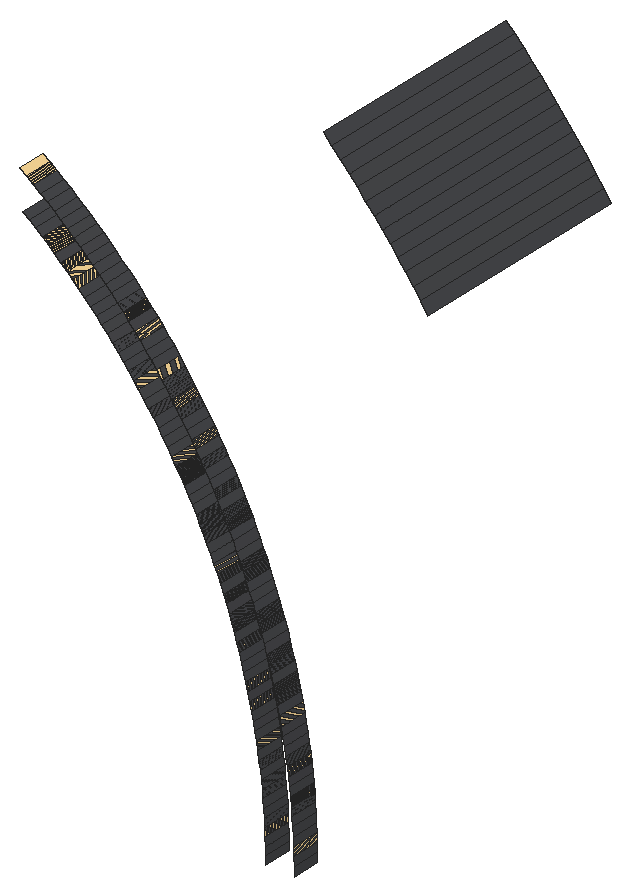
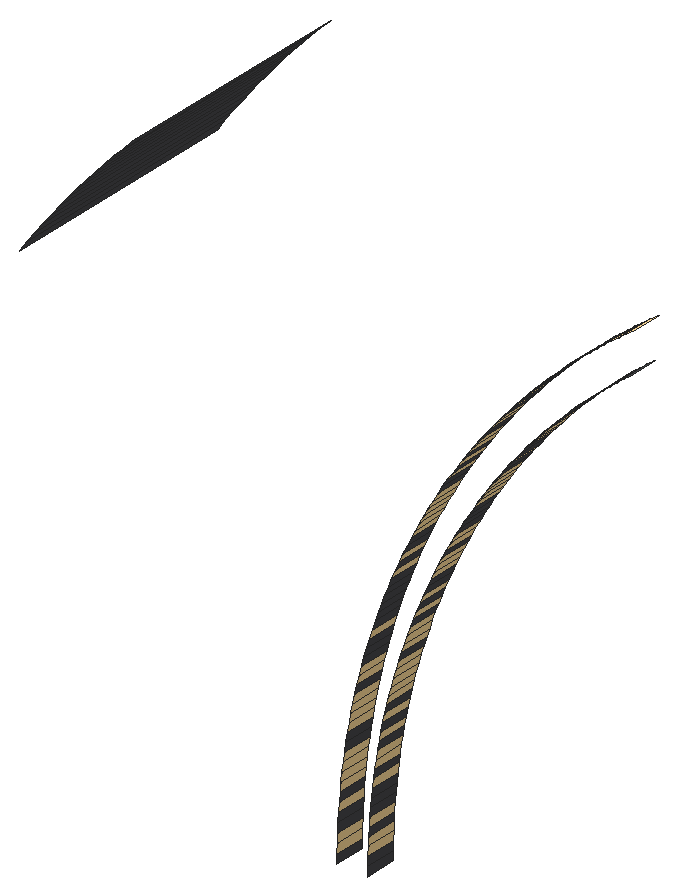
# SketchUp Ruby script. Lengths in inches.
U = 1.inch
M = Sketchup.active_model
def pt(a) = Geom::Point3d.new(a.map { |v| v * U })
def face(e, loops, mat)
  f = e.add_face(loops[0].map { |a| pt(a) })
  loops[1..].each { |l| e.add_face(l.map { |a| pt(a) }).erase! }
  f.material = f.back_material = mat if mat
  f
end
# faces: each face lists its corners as indices into pts; further lists are holes
def faces(e, pts, list, mat = nil) = list.each { |f| face(e, (f[0].is_a?(Array) ? f : [f]).map { |l| l.map { |i| pts[i] } }, mat) }
# xy, xz, yz: faces in a plane at the given z, y or x. An outline is a flat list of corners, or four numbers for a rectangle; further outlines are holes
def ring(l) = l.size == 4 ? [[l[0], l[1]], [l[2], l[1]], [l[2], l[3]], [l[0], l[3]]] : l.each_slice(2).to_a
def flat(e, list, mat, &to3) = list.each { |f| face(e, (f[0].is_a?(Array) ? f : [f]).map { |l| ring(l).map { |u, v| to3.(u, v) } }, mat) }
def xy(e, z, list, mat = nil) = flat(e, list, mat) { |x, y| [x, y, z] }
def xz(e, y, list, mat = nil) = flat(e, list, mat) { |x, z| [x, y, z] }
def yz(e, x, list, mat = nil) = flat(e, list, mat) { |y, z| [x, y, z] }
def lines(e, pts, list) = list.each { |a, b| e.add_line(pt(pts[a]), pt(pts[b])) }
# prism: a flat outline (further loops are holes) pulled along v
def prism(e, loops, v, mat = nil)
  f = face(e, loops, mat); d = Geom::Vector3d.new(v.map { |x| x * U })
  f.pushpull(f.normal.samedirection?(d) ? d.length : -d.length)
end
def box(e, o, s, mat = nil) = prism(e, [[o, [o[0] + s[0], o[1], o[2]], [o[0] + s[0], o[1] + s[1], o[2]], [o[0], o[1] + s[1], o[2]]]], [0, 0, s[2]], mat)
def at(x, y, z, deg = 0) = Geom::Transformation.translation(pt([x, y, z])) * Geom::Transformation.rotation(ORIGIN, Z_AXIS, deg.degrees)
def axes(o, x, y, z) = Geom::Transformation.new([*x, 0, *y, 0, *z, 0, *pt(o).to_a, 1])
def part(name) = M.definitions.add(name)
# library, detail: a bought-in or finely detailed component or shape, given as its bounding box
def library(name, o, s) = part(name).tap { |d| box(d.entities, o, s) }
def detail(e, o, s) = box(e.add_group.entities, o, s)
def put(e, d, t, mat = nil) = e.add_instance(d, t).tap { |i| i.material = mat if mat }
def group(e, t, mat = nil) = e.add_group.tap { |g| g.transformation = t; g.material = mat if mat }.entities
root = M.entities
M.materials.add("1432 AP 8245 TAR ROAD").color = [71, 72, 75]
M.materials.add("Outer Light").color = [251, 217, 152]
yz(root,426.5,[[95.37,410.79,96.87,411.23]],"1432 AP 8245 TAR ROAD")
yz(root,426.5,[[95.37,410.79,96.87,411.23]],"Outer Light")
yz(root,428,[[95.37,410.79,96.87,411.25]],"1432 AP 8245 TAR ROAD")
yz(root,428,[[95.37,410.79,96.87,411.25]],"Outer Light")
p = [[426.49,95.37,411.67],[426.5,95.37,411.23],[426.5,96.87,411.23],[426.49,96.87,411.67],[426.49,96.87,411.67],[426.5,96.87,411.23],
  [426.5,95.37,411.23],[426.49,95.37,411.67],[428,96.87,411.25],[427.99,96.87,411.71],[427.99,95.37,411.71],[428,95.37,411.25],
  [428,95.37,411.25],[427.99,95.37,411.71],[427.99,96.87,411.71],[428,96.87,411.25],[426.47,95.37,412.11],[426.47,96.87,412.11],
  [426.47,96.87,412.11],[426.47,95.37,412.11],[427.97,96.87,412.17],[427.97,95.37,412.17],[427.97,95.37,412.17],[427.97,96.87,412.17],
  [426.45,95.37,412.55],[426.45,96.87,412.55],[426.45,96.87,412.55],[426.45,95.37,412.55],[427.95,96.87,412.625],[427.95,95.37,412.625],
  [427.95,95.37,412.625],[427.95,96.87,412.625],[426.43,95.37,412.98],[426.43,96.87,412.98],[426.43,96.87,412.98],[426.43,95.37,412.98],
  [427.93,96.87,413.08],[427.93,95.37,413.08],[427.93,95.37,413.08],[427.93,96.87,413.08],[426.4,95.37,413.42],[426.4,96.87,413.42],
  [426.4,96.87,413.42],[426.4,95.37,413.42],[427.89,96.87,413.54],[427.89,95.37,413.54],[427.89,95.37,413.54],[427.89,96.87,413.54],
  [426.36,95.37,413.86],[426.36,96.87,413.86],[426.36,96.87,413.86],[426.36,95.37,413.86],[427.85,96.87,413.99],[427.85,95.37,413.99],
  [427.85,95.37,413.99],[427.85,96.87,413.99],[426.32,95.37,414.29],[426.32,96.87,414.29],[426.32,96.87,414.29],[426.32,95.37,414.29],
  [427.81,96.87,414.45],[427.81,95.37,414.45],[427.81,95.37,414.45],[427.81,96.87,414.45],[426.27,95.37,414.73],[426.27,96.87,414.73],
  [426.27,96.87,414.73],[426.27,95.37,414.73],[427.76,96.87,414.91],[427.76,95.37,414.91],[427.76,95.37,414.91],[427.76,96.87,414.91],
  [426.21,95.37,415.16],[426.21,96.87,415.16],[426.21,96.87,415.16],[426.21,95.37,415.16],[427.7,96.87,415.36],[427.7,95.37,415.36],
  [427.7,95.37,415.36],[427.7,96.87,415.36],[426.15,95.37,415.6],[426.15,96.87,415.6],[426.15,96.87,415.6],[426.15,95.37,415.6],
  [427.64,96.87,415.8125],[427.64,95.37,415.8125],[427.64,95.37,415.8125],[427.64,96.87,415.8125],[426.09,95.37,416.03],[426.09,96.87,416.03],
  [426.09,96.87,416.03],[426.09,95.37,416.03],[427.57,96.87,416.27],[427.57,95.37,416.27],[427.57,95.37,416.27],[427.57,96.87,416.27],
  [426.02,95.37,416.47],[426.02,96.87,416.47],[426.02,96.87,416.47],[426.02,95.37,416.47],[427.49,96.87,416.72],[427.49,95.37,416.72],
  [427.49,95.37,416.72],[427.49,96.87,416.72],[425.9375,95.37,416.9],[425.9375,96.87,416.9],[425.9375,96.87,416.9],[425.9375,95.37,416.9],
  [427.41,96.87,417.17],[427.41,95.37,417.17],[427.41,95.37,417.17],[427.41,96.87,417.17],[425.86,95.37,417.33],[425.86,96.87,417.33],
  [425.86,96.87,417.33],[425.86,95.37,417.33],[427.33,96.87,417.62],[427.33,95.37,417.62],[427.33,95.37,417.62],[427.33,96.87,417.62],
  [425.77,95.37,417.76],[425.77,96.87,417.76],[425.77,96.87,417.76],[425.77,95.37,417.76],[427.24,96.87,418.07],[427.24,95.37,418.07],
  [427.24,95.37,418.07],[427.24,96.87,418.07],[425.67,95.37,418.19],[425.67,96.87,418.19],[425.67,96.87,418.19],[425.67,95.37,418.19],
  [427.14,96.87,418.52],[427.14,95.37,418.52],[427.14,95.37,418.52],[427.14,96.87,418.52],[425.57,95.37,418.61],[425.57,96.87,418.61],
  [425.57,96.87,418.61],[425.57,95.37,418.61],[427.03,96.87,418.96],[427.03,95.37,418.96],[427.03,95.37,418.96],[427.03,96.87,418.96],
  [425.47,95.37,419.04],[425.47,96.87,419.04],[425.47,96.87,419.04],[425.47,95.37,419.04],[425.36,95.37,419.46],[425.36,96.87,419.46],
  [425.36,96.87,419.46],[425.36,95.37,419.46],[426.92,96.87,419.41],[426.92,95.37,419.41],[426.92,95.37,419.41],[426.92,96.87,419.41],
  [426.81,96.87,419.85],[426.81,95.37,419.85],[426.81,95.37,419.85],[426.81,96.87,419.85],[425.24,95.37,419.89],[425.24,96.87,419.89],
  [425.24,96.87,419.89],[425.24,95.37,419.89],[425.12,95.37,420.31],[425.12,96.87,420.31],[425.12,96.87,420.31],[425.12,95.37,420.31],
  [426.6875,96.87,420.29],[426.6875,95.37,420.29],[426.6875,95.37,420.29],[426.6875,96.87,420.29],[424.99,95.37,420.73],[424.99,96.87,420.73],
  [424.99,96.87,420.73],[424.99,95.37,420.73],[426.56,96.87,420.73],[426.56,95.37,420.73],[426.56,95.37,420.73],[426.56,96.87,420.73],
  [424.86,95.37,421.14],[424.86,96.87,421.14],[424.86,96.87,421.14],[424.86,95.37,421.14],[426.43,96.87,421.17],[426.43,95.37,421.17],
  [426.43,95.37,421.17],[426.43,96.87,421.17],[424.72,95.37,421.56],[424.72,96.87,421.56],[424.72,96.87,421.56],[424.72,95.37,421.56],
  [426.29,96.87,421.61],[426.29,95.37,421.61],[426.29,95.37,421.61],[426.29,96.87,421.61],[424.58,95.37,421.97],[424.58,96.87,421.97],
  [424.58,96.87,421.97],[424.58,95.37,421.97],[426.14,96.87,422.04],[426.14,95.37,422.04],[426.14,95.37,422.04],[426.14,96.87,422.04],
  [424.43,95.37,422.39],[424.43,96.87,422.39],[424.43,96.87,422.39],[424.43,95.37,422.39],[425.99,96.87,422.48],[425.99,95.37,422.48],
  [425.99,95.37,422.48],[425.99,96.87,422.48],[424.27,95.37,422.8],[424.27,96.87,422.8],[424.27,96.87,422.8],[424.27,95.37,422.8],
  [425.84,96.87,422.91],[425.84,95.37,422.91],[425.84,95.37,422.91],[425.84,96.87,422.91],[424.12,95.37,423.21],[424.12,96.87,423.21],
  [424.12,96.87,423.21],[424.12,95.37,423.21],[425.68,96.87,423.33],[425.68,95.37,423.33],[425.68,95.37,423.33],[425.68,96.87,423.33],
  [423.95,95.37,423.61],[423.95,96.87,423.61],[423.95,96.87,423.61],[423.95,95.37,423.61],[425.51,96.87,423.76],[425.51,95.37,423.76],
  [425.51,95.37,423.76],[425.51,96.87,423.76],[423.78,95.37,424.02],[423.78,96.87,424.02],[423.78,96.87,424.02],[423.78,95.37,424.02],
  [425.34,96.87,424.1875],[425.34,95.37,424.1875],[425.34,95.37,424.1875],[425.34,96.87,424.1875],[423.6,95.37,424.42],[423.6,96.87,424.42],
  [423.6,96.87,424.42],[423.6,95.37,424.42],[425.16,96.87,424.61],[425.16,95.37,424.61],[425.16,95.37,424.61],[425.16,96.87,424.61],
  [423.42,95.37,424.82],[423.42,96.87,424.82],[423.42,96.87,424.82],[423.42,95.37,424.82],[424.97,96.87,425.03],[424.97,95.37,425.03],
  [424.97,95.37,425.03],[424.97,96.87,425.03],[423.24,95.37,425.21],[423.24,96.87,425.21],[423.24,96.87,425.21],[423.24,95.37,425.21],
  [424.79,96.87,425.45],[424.79,95.37,425.45],[424.79,95.37,425.45],[424.79,96.87,425.45],[423.05,95.37,425.61],[423.05,96.87,425.61],
  [423.05,96.87,425.61],[423.05,95.37,425.61],[424.59,96.87,425.86],[424.59,95.37,425.86],[424.59,95.37,425.86],[424.59,96.87,425.86],
  [422.85,95.37,426],[422.85,96.87,426],[422.85,96.87,426],[422.85,95.37,426],[424.39,96.87,426.27],[424.39,95.37,426.27],
  [424.39,95.37,426.27],[424.39,96.87,426.27],[422.65,95.37,426.39],[422.65,96.87,426.39],[422.65,96.87,426.39],[422.65,95.37,426.39],
  [424.19,96.87,426.68],[424.19,95.37,426.68],[424.19,95.37,426.68],[424.19,96.87,426.68],[422.44,95.37,426.78],[422.44,96.87,426.78],
  [422.44,96.87,426.78],[422.44,95.37,426.78],[423.97,96.87,427.09],[423.97,95.37,427.09],[423.97,95.37,427.09],[423.97,96.87,427.09],
  [422.23,95.37,427.16],[422.23,96.87,427.16],[422.23,96.87,427.16],[422.23,95.37,427.16],[423.76,96.87,427.49],[423.76,95.37,427.49],
  [423.76,95.37,427.49],[423.76,96.87,427.49],[422.01,95.37,427.54],[422.01,96.87,427.54],[422.01,96.87,427.54],[422.01,95.37,427.54],
  [421.79,95.37,427.92],[421.79,96.87,427.92],[421.79,96.87,427.92],[421.79,95.37,427.92],[423.54,96.87,427.89],[423.54,95.37,427.89],
  [423.54,95.37,427.89],[423.54,96.87,427.89],[421.5625,95.37,428.3],[421.5625,96.87,428.3],[421.5625,96.87,428.3],[421.5625,95.37,428.3],
  [423.3125,96.87,428.29],[423.3125,95.37,428.29],[423.3125,95.37,428.29],[423.3125,96.87,428.29],[421.33,95.37,428.67],[421.33,96.87,428.67],
  [421.33,96.87,428.67],[421.33,95.37,428.67],[423.08,96.87,428.6875],[423.08,95.37,428.6875],[423.08,95.37,428.6875],[423.08,96.87,428.6875],
  [421.1,95.37,429.04],[421.1,96.87,429.04],[421.1,96.87,429.04],[421.1,95.37,429.04],[422.84,96.87,429.08],[422.84,95.37,429.08],
  [422.84,95.37,429.08],[422.84,96.87,429.08],[420.85,95.37,429.4],[420.85,96.87,429.4],[420.85,96.87,429.4],[420.85,95.37,429.4],
  [422.6,96.87,429.47],[422.6,95.37,429.47],[422.6,95.37,429.47],[422.6,96.87,429.47],[420.61,95.37,429.77],[420.61,96.87,429.77],
  [420.61,96.87,429.77],[420.61,95.37,429.77],[422.35,96.87,429.85],[422.35,95.37,429.85],[422.35,95.37,429.85],[422.35,96.87,429.85],
  [420.36,95.37,430.125],[420.36,96.87,430.125],[420.36,96.87,430.125],[420.36,95.37,430.125],[422.1,96.87,430.24],[422.1,95.37,430.24],
  [422.1,95.37,430.24],[422.1,96.87,430.24],[420.1,95.37,430.48],[420.1,96.87,430.48],[420.1,96.87,430.48],[420.1,95.37,430.48],
  [421.84,96.87,430.62],[421.84,95.37,430.62],[421.84,95.37,430.62],[421.84,96.87,430.62],[419.84,95.37,430.84],[419.84,96.87,430.84],
  [419.84,96.87,430.84],[419.84,95.37,430.84],[421.58,96.87,430.99],[421.58,95.37,430.99],[421.58,95.37,430.99],[421.58,96.87,430.99],
  [419.58,95.37,431.1875],[419.58,96.87,431.1875],[419.58,96.87,431.1875],[419.58,95.37,431.1875],[421.32,96.87,431.36],[421.32,95.37,431.36],
  [421.32,95.37,431.36],[421.32,96.87,431.36],[419.31,95.37,431.53],[419.31,96.87,431.53],[419.31,96.87,431.53],[419.31,95.37,431.53],
  [421.04,96.87,431.73],[421.04,95.37,431.73],[421.04,95.37,431.73],[421.04,96.87,431.73],[419.03,95.37,431.875],[419.03,96.87,431.875],
  [419.03,96.87,431.875],[419.03,95.37,431.875],[420.77,96.87,432.1],[420.77,95.37,432.1],[420.77,95.37,432.1],[420.77,96.87,432.1],
  [418.76,95.37,432.21],[418.76,96.87,432.21],[418.76,96.87,432.21],[418.76,95.37,432.21],[420.49,96.87,432.46],[420.49,95.37,432.46],
  [420.49,95.37,432.46],[420.49,96.87,432.46],[418.47,95.37,432.55],[418.47,96.87,432.55],[418.47,96.87,432.55],[418.47,95.37,432.55],
  [418.1875,95.37,432.88],[418.1875,96.87,432.88],[418.1875,96.87,432.88],[418.1875,95.37,432.88],[420.2,96.87,432.82],[420.2,95.37,432.82],
  [420.2,95.37,432.82],[420.2,96.87,432.82],[419.91,96.87,433.17],[419.91,95.37,433.17],[419.91,95.37,433.17],[419.91,96.87,433.17],
  [417.9,95.37,433.21],[417.9,96.87,433.21],[417.9,96.87,433.21],[417.9,95.37,433.21],[417.6,95.37,433.53],[417.6,96.87,433.53],
  [417.6,96.87,433.53],[417.6,95.37,433.53],[419.61,96.87,433.52],[419.61,95.37,433.52],[419.61,95.37,433.52],[419.61,96.87,433.52],
  [417.3,95.37,433.85],[417.3,96.87,433.85],[417.3,96.87,433.85],[417.3,95.37,433.85],[419.3125,96.87,433.87],[419.3125,95.37,433.87],
  [419.3125,95.37,433.87],[419.3125,96.87,433.87],[417,95.37,434.17],[417,96.87,434.17],[417,96.87,434.17],[417,95.37,434.17],
  [419.01,96.87,434.21],[419.01,95.37,434.21],[419.01,95.37,434.21],[419.01,96.87,434.21],[416.6875,95.37,434.48],[416.6875,96.87,434.48],
  [416.6875,96.87,434.48],[416.6875,95.37,434.48],[418.7,96.87,434.55],[418.7,95.37,434.55],[418.7,95.37,434.55],[418.7,96.87,434.55],
  [416.375,95.37,434.79],[416.375,96.87,434.79],[416.375,96.87,434.79],[416.375,95.37,434.79],[418.39,96.87,434.88],[418.39,95.37,434.88],
  [418.39,95.37,434.88],[418.39,96.87,434.88],[416.06,95.37,435.09],[416.06,96.87,435.09],[416.06,96.87,435.09],[416.06,95.37,435.09],
  [418.07,96.87,435.21],[418.07,95.37,435.21],[418.07,95.37,435.21],[418.07,96.87,435.21],[415.74,95.37,435.39],[415.74,96.87,435.39],
  [415.74,96.87,435.39],[415.74,95.37,435.39],[417.75,96.87,435.54],[417.75,95.37,435.54],[417.75,95.37,435.54],[417.75,96.87,435.54],
  [415.42,95.37,435.6875],[415.42,96.87,435.6875],[415.42,96.87,435.6875],[415.42,95.37,435.6875],[417.42,96.87,435.86],[417.42,95.37,435.86],
  [417.42,95.37,435.86],[417.42,96.87,435.86],[415.09,95.37,435.98],[415.09,96.87,435.98],[415.09,96.87,435.98],[415.09,95.37,435.98],
  [417.09,96.87,436.18],[417.09,95.37,436.18],[417.09,95.37,436.18],[417.09,96.87,436.18],[414.76,95.37,436.27],[414.76,96.87,436.27],
  [414.76,96.87,436.27],[414.76,95.37,436.27],[416.76,96.87,436.49],[416.76,95.37,436.49],[416.76,95.37,436.49],[416.76,96.87,436.49],
  [414.42,95.37,436.55],[414.42,96.87,436.55],[414.42,96.87,436.55],[414.42,95.37,436.55],[414.08,95.37,436.83],[414.08,96.87,436.83],
  [414.08,96.87,436.83],[414.08,95.37,436.83],[416.42,96.87,436.8],[416.42,95.37,436.8],[416.42,95.37,436.8],[416.42,96.87,436.8],
  [413.74,95.37,437.1],[413.74,96.87,437.1],[413.74,96.87,437.1],[413.74,95.37,437.1],[416.08,96.87,437.11],[416.08,95.37,437.11],
  [416.08,95.37,437.11],[416.08,96.87,437.11],[415.73,96.87,437.41],[415.73,95.37,437.41],[415.73,95.37,437.41],[415.73,96.87,437.41],
  [415.38,96.87,437.7],[415.38,95.37,437.7],[415.38,95.37,437.7],[415.38,96.87,437.7],[415.03,96.87,437.99],[415.03,95.37,437.99],
  [415.03,95.37,437.99],[415.03,96.87,437.99],[414.67,96.87,438.28],[414.67,95.37,438.28],[414.67,95.37,438.28],[414.67,96.87,438.28],
  [414.31,96.87,438.56],[414.31,95.37,438.56],[414.31,95.37,438.56],[414.31,96.87,438.56],[413.94,96.87,438.84],[413.94,95.37,438.84],
  [413.94,95.37,438.84],[413.94,96.87,438.84],[413.57,96.87,439.11],[413.57,95.37,439.11],[435.03,107.37,439.68],[434.65,107.37,440.23],
  [434.65,95.37,440.23],[435.03,95.37,439.68],[434.26,107.37,440.77],[434.26,95.37,440.77],[433.86,107.37,441.31],[433.86,95.37,441.31],
  [433.46,107.37,441.84],[433.46,95.37,441.84],[433.05,107.37,442.37],[433.05,95.37,442.37],[432.63,107.37,442.89],[432.63,95.37,442.89],
  [432.21,107.37,443.4],[432.21,95.37,443.4],[431.78,107.37,443.91],[431.78,95.37,443.91],[431.34,107.37,444.42],[431.34,95.37,444.42],
  [430.9,107.37,444.92],[430.9,95.37,444.92],[430.45,107.37,445.41],[430.45,95.37,445.41],[429.99,107.37,445.9],[429.99,95.37,445.9],
  [429.53,107.37,446.38],[429.53,95.37,446.38]]
faces(root,p,[[0,1,2,3],[12,13,14,15],[16,0,3,17],[13,22,23,14],[24,16,17,25],[22,30,31,23],[32,24,25,33],[30,38,39,31],
  [40,32,33,41],[38,46,47,39],[48,40,41,49],[46,54,55,47],[56,48,49,57],[54,62,63,55],[64,56,57,65],[62,70,71,63],
  [72,64,65,73],[70,78,79,71],[80,72,73,81],[78,86,87,79],[88,80,81,89],[86,94,95,87],[96,88,89,97],[94,102,103,95],
  [104,96,97,105],[102,110,111,103],[112,104,105,113],[110,118,119,111],[120,112,113,121],[118,126,127,119],[128,120,121,129],[126,134,135,127],
  [136,128,129,137],[134,142,143,135],[144,136,137,145],[148,144,145,149],[142,154,155,143],[154,158,159,155],[160,148,149,161],[164,160,161,165],
  [158,170,171,159],[172,164,165,173],[170,178,179,171],[180,172,173,181],[178,186,187,179],[188,180,181,189],[186,194,195,187],[196,188,189,197],
  [194,202,203,195],[204,196,197,205],[202,210,211,203],[212,204,205,213],[210,218,219,211],[220,212,213,221],[218,226,227,219],[228,220,221,229],
  [226,234,235,227],[236,228,229,237],[234,242,243,235],[244,236,237,245],[242,250,251,243],[252,244,245,253],[250,258,259,251],[260,252,253,261],
  [258,266,267,259],[268,260,261,269],[266,274,275,267],[276,268,269,277],[274,282,283,275],[284,276,277,285],[282,290,291,283],[292,284,285,293],
  [290,298,299,291],[300,292,293,301],[298,306,307,299],[308,300,301,309],[312,308,309,313],[306,318,319,307],[320,312,313,321],[318,326,327,319],
  [328,320,321,329],[326,334,335,327],[336,328,329,337],[334,342,343,335],[344,336,337,345],[342,350,351,343],[352,344,345,353],[350,358,359,351],
  [360,352,353,361],[358,366,367,359],[368,360,361,369],[366,374,375,367],[376,368,369,377],[374,382,383,375],[384,376,377,385],[382,390,391,383],
  [392,384,385,393],[390,398,399,391],[400,392,393,401],[398,406,407,399],[408,400,401,409],[406,414,415,407],[416,408,409,417],[420,416,417,421],
  [414,426,427,415],[426,430,431,427],[432,420,421,433],[436,432,433,437],[430,442,443,431],[444,436,437,445],[442,450,451,443],[452,444,445,453],
  [450,458,459,451],[460,452,453,461],[458,466,467,459],[468,460,461,469],[466,474,475,467],[476,468,469,477],[474,482,483,475],[484,476,477,485],
  [482,490,491,483],[492,484,485,493],[490,498,499,491],[500,492,493,501],[498,506,507,499],[508,500,501,509],[506,514,515,507],[516,508,509,517],
  [520,516,517,521],[514,526,527,515],[528,520,521,529],[526,534,535,527],[534,538,539,535],[538,542,543,539],[542,546,547,543],[546,550,551,547],
  [550,554,555,551],[554,558,559,555],[562,563,564,565],[563,566,567,564],[566,568,569,567],[568,570,571,569],[570,572,573,571],[572,574,575,573],
  [574,576,577,575],[576,578,579,577],[578,580,581,579],[580,582,583,581],[582,584,585,583],[584,586,587,585],[586,588,589,587]],"1432 AP 8245 TAR ROAD")
faces(root,p,[[4,5,6,7],[8,9,10,11],[18,4,7,19],[9,20,21,10],[26,18,19,27],[20,28,29,21],[34,26,27,35],[28,36,37,29],
  [42,34,35,43],[36,44,45,37],[50,42,43,51],[44,52,53,45],[58,50,51,59],[52,60,61,53],[66,58,59,67],[60,68,69,61],
  [74,66,67,75],[68,76,77,69],[82,74,75,83],[76,84,85,77],[90,82,83,91],[84,92,93,85],[98,90,91,99],[92,100,101,93],
  [106,98,99,107],[100,108,109,101],[114,106,107,115],[108,116,117,109],[122,114,115,123],[116,124,125,117],[130,122,123,131],[124,132,133,125],
  [138,130,131,139],[132,140,141,133],[146,138,139,147],[150,146,147,151],[140,152,153,141],[152,156,157,153],[162,150,151,163],[166,162,163,167],
  [156,168,169,157],[174,166,167,175],[168,176,177,169],[182,174,175,183],[176,184,185,177],[190,182,183,191],[184,192,193,185],[198,190,191,199],
  [192,200,201,193],[206,198,199,207],[200,208,209,201],[214,206,207,215],[208,216,217,209],[222,214,215,223],[216,224,225,217],[230,222,223,231],
  [224,232,233,225],[238,230,231,239],[232,240,241,233],[246,238,239,247],[240,248,249,241],[254,246,247,255],[248,256,257,249],[262,254,255,263],
  [256,264,265,257],[270,262,263,271],[264,272,273,265],[278,270,271,279],[272,280,281,273],[286,278,279,287],[280,288,289,281],[294,286,287,295],
  [288,296,297,289],[302,294,295,303],[296,304,305,297],[310,302,303,311],[314,310,311,315],[304,316,317,305],[322,314,315,323],[316,324,325,317],
  [330,322,323,331],[324,332,333,325],[338,330,331,339],[332,340,341,333],[346,338,339,347],[340,348,349,341],[354,346,347,355],[348,356,357,349],
  [362,354,355,363],[356,364,365,357],[370,362,363,371],[364,372,373,365],[378,370,371,379],[372,380,381,373],[386,378,379,387],[380,388,389,381],
  [394,386,387,395],[388,396,397,389],[402,394,395,403],[396,404,405,397],[410,402,403,411],[404,412,413,405],[418,410,411,419],[422,418,419,423],
  [412,424,425,413],[424,428,429,425],[434,422,423,435],[438,434,435,439],[428,440,441,429],[446,438,439,447],[440,448,449,441],[454,446,447,455],
  [448,456,457,449],[462,454,455,463],[456,464,465,457],[470,462,463,471],[464,472,473,465],[478,470,471,479],[472,480,481,473],[486,478,479,487],
  [480,488,489,481],[494,486,487,495],[488,496,497,489],[502,494,495,503],[496,504,505,497],[510,502,503,511],[504,512,513,505],[518,510,511,519],
  [522,518,519,523],[512,524,525,513],[530,522,523,531],[524,532,533,525],[532,536,537,533],[536,540,541,537],[540,544,545,541],[544,548,549,545],
  [548,552,553,549],[552,556,557,553],[556,560,561,557]],"Outer Light")
